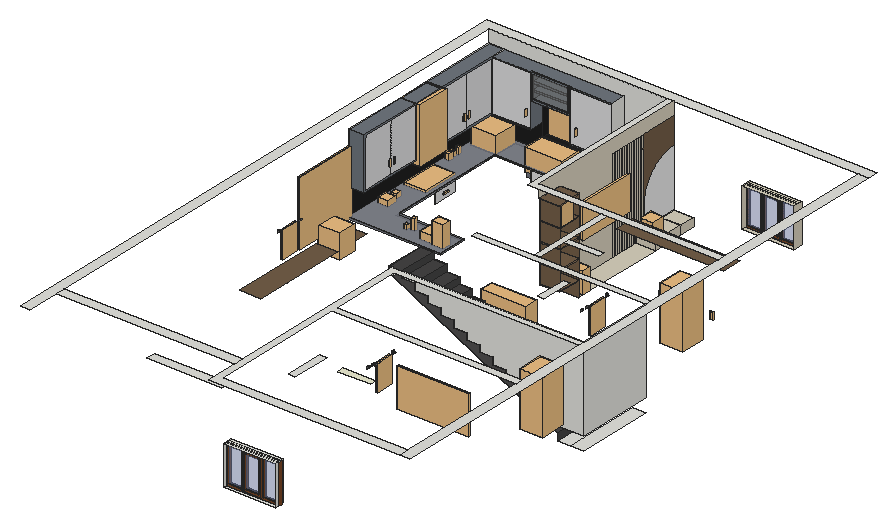
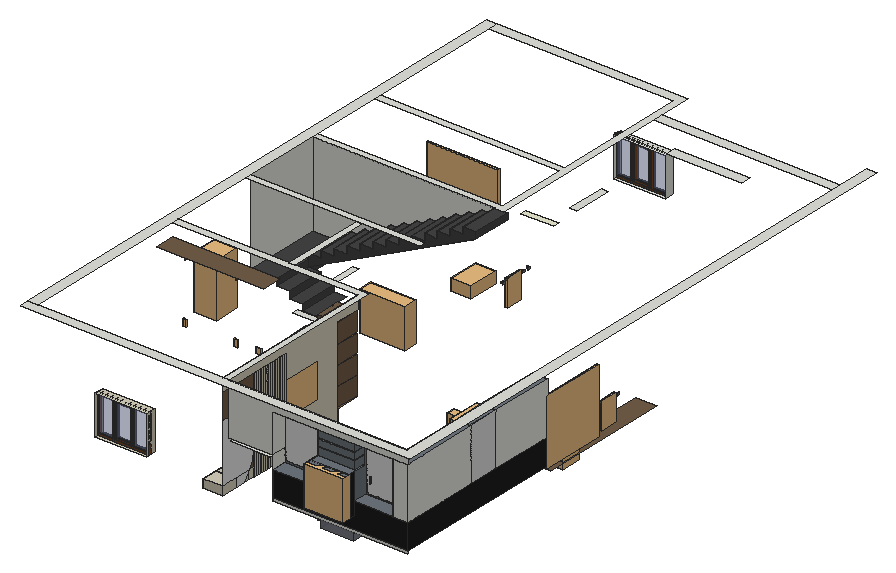
# SketchUp Ruby script. Lengths in inches.
U = 1.inch
M = Sketchup.active_model
def pt(a) = Geom::Point3d.new(a.map { |v| v * U })
def face(e, loops, mat)
  f = e.add_face(loops[0].map { |a| pt(a) })
  loops[1..].each { |l| e.add_face(l.map { |a| pt(a) }).erase! }
  f.material = f.back_material = mat if mat
  f
end
# faces: each face lists its corners as indices into pts; further lists are holes
def faces(e, pts, list, mat = nil) = list.each { |f| face(e, (f[0].is_a?(Array) ? f : [f]).map { |l| l.map { |i| pts[i] } }, mat) }
# xy, xz, yz: faces in a plane at the given z, y or x. An outline is a flat list of corners, or four numbers for a rectangle; further outlines are holes
def ring(l) = l.size == 4 ? [[l[0], l[1]], [l[2], l[1]], [l[2], l[3]], [l[0], l[3]]] : l.each_slice(2).to_a
def flat(e, list, mat, &to3) = list.each { |f| face(e, (f[0].is_a?(Array) ? f : [f]).map { |l| ring(l).map { |u, v| to3.(u, v) } }, mat) }
def xy(e, z, list, mat = nil) = flat(e, list, mat) { |x, y| [x, y, z] }
def xz(e, y, list, mat = nil) = flat(e, list, mat) { |x, z| [x, y, z] }
def yz(e, x, list, mat = nil) = flat(e, list, mat) { |y, z| [x, y, z] }
def lines(e, pts, list) = list.each { |a, b| e.add_line(pt(pts[a]), pt(pts[b])) }
# prism: a flat outline (further loops are holes) pulled along v
def prism(e, loops, v, mat = nil)
  f = face(e, loops, mat); d = Geom::Vector3d.new(v.map { |x| x * U })
  f.pushpull(f.normal.samedirection?(d) ? d.length : -d.length)
end
def box(e, o, s, mat = nil) = prism(e, [[o, [o[0] + s[0], o[1], o[2]], [o[0] + s[0], o[1] + s[1], o[2]], [o[0], o[1] + s[1], o[2]]]], [0, 0, s[2]], mat)
def at(x, y, z, deg = 0) = Geom::Transformation.translation(pt([x, y, z])) * Geom::Transformation.rotation(ORIGIN, Z_AXIS, deg.degrees)
def axes(o, x, y, z) = Geom::Transformation.new([*x, 0, *y, 0, *z, 0, *pt(o).to_a, 1])
def part(name) = M.definitions.add(name)
# library, detail: a bought-in or finely detailed component or shape, given as its bounding box
def library(name, o, s) = part(name).tap { |d| box(d.entities, o, s) }
def detail(e, o, s) = box(e.add_group.entities, o, s)
def put(e, d, t, mat = nil) = e.add_instance(d, t).tap { |i| i.material = mat if mat }
def group(e, t, mat = nil) = e.add_group.tap { |g| g.transformation = t; g.material = mat if mat }.entities
root = M.entities
M.materials.add("0746 AP 7715 LUMINOUS").color = [235, 235, 209]
M.materials.add("1442 AP K091 Frozen Zanskar-N").color = [220, 220, 221]
M.materials.add("1446 AP 8255 STONE PATH").color = [111, 118, 125]
M.materials.add("1689 AP 8482 GREY BUCK").color = [214, 207, 188]
M.materials.add("CROMADO1").color = [109, 109, 109]
M.materials.add("Granite Padang Light 150cm").color = [116, 119, 128]
M.materials["Granite Padang Light 150cm"].alpha = 0.92
M.materials.add("Tiles Marble Black 01 160cm").color = [32, 32, 32]
M.materials.add("Wood Pecan 33-21 150cm").color = [115, 94, 72]
M.materials.add("Wood Walnut 33-38 100cm").color = [48, 31, 12]
M.materials.add("[Granite Dark Gray]").color = [69, 68, 68]
M.materials.add("[Mirror 02]").color = [229, 229, 229]
M.materials.add("[Translucent Glass Gray]").color = [128, 128, 128]
M.materials["[Translucent Glass Gray]"].alpha = 0.5
M.materials.add("[Translucent Glass Sky Reflection]1").color = [126, 138, 183]
M.materials["[Translucent Glass Sky Reflection]1"].alpha = 0.52
M.materials.add("[Wood Veneer 01]").color = [120, 70, 37]
M.materials.add("w-001").color = [255, 255, 255]
c1 = library("1-VASEFLEURS CLC2",[-4.93,-4.36,0],[9.88,8.02,19.93])
c2 = library("3-EVIER M60 CLC2\#1",[-8.86,-8.86,-7.51],[17.72,19.62,22.02])
c3 = library("1-POIGNEE CLC2\#1",[-3.03,-0.375,0],[6.06,0.75,1.42])
c4 = library("1-POIGNEE CLC2\#2",[-3.03,-0.375,0],[6.06,0.75,1.42])
c5 = library("4",[-16.3,-15.81,0],[32.6,31.62,37.8])
c6 = library("4-EVIER M80 CLC2",[-16.92,-9.84,-5.67],[33.86,19.68,19.96])
c7 = library("Towel",[0,0,0],[10.6875,1.92,14.5625])
c8 = library("MOROCCAN+WASH+BASIN",[-11.85,-9.27,0.39],[28.27,18.54,10.92])
c9 = library("HUDSON+mirror",[-29.92,-0.89,23.77],[59.84,1.78,59.94])
c10 = library("1-MICRO H40 CLC2",[0,-1.46,0],[23.5,21.66,15.63])
c11 = library("1-PNGFRUITS CLC2",[-5.8,-5.64,-0.15],[11.3,11.71,6.42])
c12 = part("beroom window")
xy(c12.entities,-0.21,[[0,2.95,48.51,5.71]],"[Wood Veneer 01]")
xy(c12.entities,0.95,[[16.09,2.17,32.42,2.95]],"[Wood Veneer 01]")
xy(c12.entities,1.1875,[[1.44,2.95,14.41,4.33],[16.33,2.95,32.18,4.92],[34.1,2.95,47.07,4.33],[1.44,4.33,14.41,5.71],[34.1,4.33,47.07,5.71],
  [16.33,4.92,32.18,5.71]],"[Wood Veneer 01]")
xy(c12.entities,2.58,[[17.77,2.17,30.74,3.54],[17.77,3.54,30.74,4.92]],"[Wood Veneer 01]")
xy(c12.entities,29.62,[[17.77,2.17,30.74,3.54],[17.77,3.54,30.74,4.92]],"[Wood Veneer 01]")
xy(c12.entities,31.02,[[1.44,2.95,14.41,4.33],[16.33,2.95,32.18,4.92],[34.1,2.95,47.07,4.33],[1.44,4.33,14.41,5.71],[34.1,4.33,47.07,5.71],
  [16.33,4.92,32.18,5.71]],"[Wood Veneer 01]")
xy(c12.entities,31.25,[[16.09,2.17,32.42,2.95]],"[Wood Veneer 01]")
xy(c12.entities,32.42,[[0,2.95,48.51,5.71]],"[Wood Veneer 01]")
xz(c12.entities,2.17,[[[16.09,0.95,32.42,31.25],[17.77,2.58,30.74,29.62]]],"[Wood Veneer 01]")
xz(c12.entities,2.95,[[[0,-0.21,48.51,32.42],[16.33,1.1875,32.18,31.02],[1.44,1.1875,14.41,31.02],[34.1,1.1875,47.07,31.02]]],"[Wood Veneer 01]")
xz(c12.entities,3.54,[[17.77,2.58,30.74,29.62]],"[Translucent Glass Sky Reflection]1")
xz(c12.entities,4.33,[[1.44,1.1875,14.41,31.02],[34.1,1.1875,47.07,31.02]],"[Translucent Glass Sky Reflection]1")
xz(c12.entities,4.92,[[[16.33,1.1875,32.18,31.02],[17.77,2.58,30.74,29.62]]],"[Wood Veneer 01]")
xz(c12.entities,5.71,[[[0,-0.21,48.51,32.42],[16.33,1.1875,32.18,31.02],[1.44,1.1875,14.41,31.02],[34.1,1.1875,47.07,31.02]]],"[Wood Veneer 01]")
yz(c12.entities,0,[[2.95,-0.21,5.71,32.42]],"[Wood Veneer 01]")
yz(c12.entities,1.44,[[2.95,1.1875,4.33,31.02],[4.33,1.1875,5.71,31.02]],"[Wood Veneer 01]")
yz(c12.entities,14.41,[[2.95,1.1875,4.33,31.02],[4.33,1.1875,5.71,31.02]],"[Wood Veneer 01]")
yz(c12.entities,16.09,[[2.17,0.95,2.95,31.25]],"[Wood Veneer 01]")
yz(c12.entities,16.33,[[2.95,1.1875,4.92,31.02],[4.92,1.1875,5.71,31.02]],"[Wood Veneer 01]")
yz(c12.entities,17.77,[[2.17,2.58,3.54,29.62],[3.54,2.58,4.92,29.62]],"[Wood Veneer 01]")
yz(c12.entities,30.74,[[2.17,2.58,3.54,29.62],[3.54,2.58,4.92,29.62]],"[Wood Veneer 01]")
yz(c12.entities,32.18,[[2.95,1.1875,4.92,31.02],[4.92,1.1875,5.71,31.02]],"[Wood Veneer 01]")
yz(c12.entities,32.42,[[2.17,0.95,2.95,31.25]],"[Wood Veneer 01]")
yz(c12.entities,34.1,[[2.95,1.1875,4.33,31.02],[4.33,1.1875,5.71,31.02]],"[Wood Veneer 01]")
yz(c12.entities,47.07,[[2.95,1.1875,4.33,31.02],[4.33,1.1875,5.71,31.02]],"[Wood Veneer 01]")
yz(c12.entities,48.51,[[2.95,-0.21,5.71,32.42]],"[Wood Veneer 01]")
g1 = group(c12.entities,at(16.61,2.17,13.98),"w-001")
xy(g1,0,[[0.12,-2.17,0.53,-1.77]])
xy(g1,1.57,[[0,-0.39,0.65,0]])
xy(g1,2.1,[[0.12,-1.77,0.53,-0.39]])
xy(g1,2.5625,[[0.12,-2.17,0.53,-0.39]])
xy(g1,3.09,[[0,-0.39,0.65,0]])
xz(g1,-2.17,[[0.12,0,0.53,2.5625]])
xz(g1,-1.77,[[0.12,0,0.53,2.1]])
xz(g1,-0.39,[[[0,1.57,0.65,3.09],[0.12,2.1,0.53,2.5625]]])
xz(g1,0,[[0,1.57,0.65,3.09]])
yz(g1,0,[[-0.39,1.57,0,3.09]])
yz(g1,0.12,[[-2.17,0,-2.17,2.5625,-0.39,2.5625,-0.39,2.1,-1.77,2.1,-1.77,0]])
yz(g1,0.53,[[-2.17,0,-1.77,0,-1.77,2.1,-0.39,2.1,-0.39,2.5625,-2.17,2.5625]])
yz(g1,0.65,[[-0.39,1.57,0,3.09]])
c13 = library("16-PRODUITS CUISINE CLC2",[-2.49,-2.49,0],[4.98,4.98,4.3])
c14 = library("10-PRODUITS CUISINE CLC2",[-4.7,-4.62,0],[9.45,9.45,4.72])
c15 = library("3-PRODUITS CUISINE CLC2",[-1.54,-1.54,0],[3.08,3.08,10.36])
c16 = library("13-PRODUITS CUISINE CLC2",[-1.97,-1.97,0],[3.94,3.94,3.9375])
c17 = library("20-PRODUITS CUISINE CLC2",[-1.38,-1.38,0],[2.76,2.76,3.9375])
c18 = library("15-PRODUITS CUISINE CLC2",[-1.94,-2.15,0],[3.93,3.94,5.51])
c19 = library("22-PRODUITS CUISINE CLC2",[-2.93,-2.91,0],[5.9,5.9,2.76])
c20 = library("7-TABLE DE CUISSON CLC2",[-16.93,-10.04,0.13],[33.86,20.08,1.97])
c21 = library("23-PRODUITS CUISINE CLC2",[-4.92,-4.92,-0.18],[9.84,9.84,0.98])
c22 = library("11-PRODUITS CUISINE CLC2",[-1.48,-1.48,0],[2.96,2.96,6.14])
c23 = library("deca slim quadrada",[0,0,0],[0.79,5.12,5.12])
c24 = library("Bathroom vanity",[0,-2.21,0],[70.12,25.94,41.93])
c25 = library("Kitchen Window",[0,0,0],[58.5625,13.48,48])
c26 = library("Shower Raindance Connect",[1.71,-11.67,0],[20.76,23.22,49.85])
c27 = library("Ribe+Handles+timber",[52.85,54.46,0],[0.74,3.05,6.14])
c28 = library("Flat screen television",[-21.7,-0.05,0],[43.4,2.31,25.36])
c29 = part("Group\#170")
g2 = group(c29.entities,at(0.87,1.79,0.87))
box(g2,[-0.87,-0.39,-0.87],[1.74,0.39,1.74],"CROMADO1")
g3 = group(c29.entities,at(0.87,1.79,0.87))
prism(g3,[[[-0.1875,-1.42,1.39],[-0.1875,-1.42,0.1875],[-0.1875,-0.39,0.1875],[-0.1875,-0.39,-0.1875],[-0.1875,-1.79,-0.1875],[-0.1875,-1.79,1.39]]],[0.375,0,0],"CROMADO1")
c30 = part("Group\#166")
xy(c30.entities,0,[[-6.57,-0.87,-6.59,-0.85,-6.59,0.85,-6.57,0.87,-4.87,0.87,-4.85,0.85,-4.85,-0.85,-4.87,-0.87],[16.68,-0.87,16.66,-0.85,16.66,0.85,16.68,0.87,18.38,0.87,18.4,0.85,18.4,-0.85,18.38,-0.87]],"CROMADO1")
xy(c30.entities,0.39,[[[-6.57,-0.87,-4.87,-0.87,-4.85,-0.85,-4.85,0.85,-4.87,0.87,-6.57,0.87,-6.59,0.85,-6.59,-0.85],[-5.91,-0.1875,-5.53,0.1875]],[[16.68,-0.87,18.38,-0.87,18.4,-0.85,18.4,0.85,18.38,0.87,16.68,0.87,16.66,0.85,16.66,-0.85],[17.34,-0.1875,17.72,0.1875]]],"CROMADO1")
xy(c30.entities,2.15,[[-5.53,-0.1875,17.34,0.1875]],"CROMADO1")
xy(c30.entities,2.52,[[-5.91,-0.1875,17.72,0.1875]],"CROMADO1")
xz(c30.entities,-0.87,[[-6.57,0,-4.87,0.39],[16.68,0,18.38,0.39]],"CROMADO1")
xz(c30.entities,-0.1875,[[-5.91,0.39,-5.53,0.39,-5.53,2.15,17.34,2.15,17.34,0.39,17.72,0.39,17.72,2.52,-5.91,2.52]])
xz(c30.entities,0.1875,[[-5.91,0.39,-5.91,2.52,17.72,2.52,17.72,0.39,17.34,0.39,17.34,2.15,-5.53,2.15,-5.53,0.39]],"CROMADO1")
xz(c30.entities,0.87,[[-6.57,0,-4.87,0.39],[16.68,0,18.38,0.39]],"CROMADO1")
yz(c30.entities,-6.59,[[-0.85,0,0.85,0.39]],"CROMADO1")
yz(c30.entities,-5.91,[[-0.1875,0.39,0.1875,2.52]],"CROMADO1")
yz(c30.entities,-5.53,[[-0.1875,0.39,0.1875,2.15]],"CROMADO1")
yz(c30.entities,-4.85,[[-0.85,0,0.85,0.39]],"CROMADO1")
yz(c30.entities,16.66,[[-0.85,0,0.85,0.39]],"CROMADO1")
yz(c30.entities,17.34,[[-0.1875,0.39,0.1875,2.15]],"CROMADO1")
yz(c30.entities,17.72,[[-0.1875,0.39,0.1875,2.52]],"CROMADO1")
yz(c30.entities,18.4,[[-0.85,0,0.85,0.39]],"CROMADO1")
p = [[-6.57,-0.87,0.39],[-6.59,-0.85,0.39],[-6.59,-0.85,0],[-6.57,-0.87,0],[-4.85,-0.85,0.39],[-4.87,-0.87,0.39],
  [-4.87,-0.87,0],[-4.85,-0.85,0],[16.68,-0.87,0.39],[16.66,-0.85,0.39],[16.66,-0.85,0],[16.68,-0.87,0],
  [18.4,-0.85,0],[18.4,-0.85,0.39],[18.38,-0.87,0.39],[18.38,-0.87,0],[-6.57,0.87,0],[-6.59,0.85,0],
  [-6.59,0.85,0.39],[-6.57,0.87,0.39],[-4.85,0.85,0],[-4.87,0.87,0],[-4.87,0.87,0.39],[-4.85,0.85,0.39],
  [16.68,0.87,0.39],[16.68,0.87,0],[16.66,0.85,0],[16.66,0.85,0.39],[18.38,0.87,0],[18.38,0.87,0.39],
  [18.4,0.85,0.39],[18.4,0.85,0]]
faces(c30.entities,p,[[0,1,2,3],[4,5,6,7],[8,9,10,11],[12,13,14,15],[16,17,18,19],[20,21,22,23],[24,25,26,27],[28,29,30,31]])
c31 = library("5-HOTTE ASPIRANTE CLC2",[-15.16,-17.72,-0.29],[30.34,17.72,30.09])
c32 = library("Dekoracija24",[-23.93,-1.04,68.5625],[48.15,1.24,26.11])
c33 = library("1-POIGNEE CLC2\#3",[-3.03,-0.375,0],[6.06,0.75,1.42])
c34 = library("6-VASEFLEURS CLC2",[-8.63,-6.29,0],[14.28,12.79,17.02])
xy(root,22,[[180,399,198,487],[179.5,459,180,460],[179.5,461,180,462],[179.5,463,180,464],[179.5,465,180,466],
  [179.5,467,180,468],[179.5,469,180,470],[179.5,471,180,472],[179.5,473,180,474],[179.5,475,180,476],
  [179.5,477,180,478],[179.5,479,180,480],[179.5,481,180,482],[179.5,483,180,484],[179.5,485,180,486],
  [179.5,487,180,488],[180,487,198,495],[179.5,489,180,490],[179.5,491,180,492],[179.5,493,180,494],
  [180,495,198,501.67],[180,501.67,198,516.33],[180,516.33,198,531]],"1689 AP 8482 GREY BUCK")
xy(root,23.7,[[32.7,438.9,33,461.4],[66.97,507,100.33,507.3]],"1442 AP K091 Frozen Zanskar-N")
xy(root,24,[[32.7,438.9,32.8,461.4],[32.8,438.9,33,461.4],[66.97,507,100.33,507.3]],"1442 AP K091 Frozen Zanskar-N")
xy(root,24,[[61.45,509.36,92.2,527.24]],"Granite Padang Light 150cm")
xy(root,24,[[291,249,303,285]],"[Granite Dark Gray]")
xy(root,29,[[28.39,273.63,28.6875,273.93],[28.39,333.67,28.6875,333.97]],"Wood Pecan 33-21 150cm")
xy(root,30,[[327,213,339,249],[339,213,351,285]])
xy(root,30,[[180,487,198,501.67],[180,501.67,198,516.33],[180,516.33,198,531]],"1689 AP 8482 GREY BUCK")
xy(root,30,[[[9,242.61,28.6875,364.7],[19.02,331.45,16.86,331.97,14.9,333.03,13.29,334.5625,12.125,336.46,11.49,338.59,11.43,340.82,11.95,342.98,13.01,344.9375,14.55,346.55,16.44,347.71,18.58,348.35,20.8,348.4,22.96,347.88,24.92,346.82,26.53,345.29,27.7,343.39,28.33,341.26,28.39,339.04,27.87,336.87,26.81,334.92,25.27,333.3,23.375,332.14,21.24,331.51]]],"Wood Pecan 33-21 150cm")
xy(root,30,[[303,249,315,285]],"[Granite Dark Gray]")
xy(root,34,[[9,367,95,369],[93,369,95,393],[62.7,392.7,62.7,393,33,393,33,415.8,32.7,415.8,32.7,416.1,33,416.1,33,438.6,32.7,438.6,32.7,438.9,33,438.9,33,461.4,32.7,461.4,32.7,461.7,33,461.7,33,484.2,32.7,484.2,32.7,484.5,33,484.5,33,507,66.67,507,66.67,507.3,66.97,507.3,66.97,507,100.33,507,100.33,507.3,100.63,507.3,100.63,507,134,507,134,505,35,505,35,395,95,395,95,393,63,393,63,392.7]],"Granite Padang Light 150cm")
xy(root,36,[[188,0,236,9]])
xy(root,36,[[243,531,291,540]],"1689 AP 8482 GREY BUCK")
xy(root,36,[[[9,367,95,367,95,395,35,395,35,505,134,505,134,531,9,531],[61.45,509.36,92.2,527.24]]],"Granite Padang Light 150cm")
xy(root,36,[[180,376,198,398]],"Wood Pecan 33-21 150cm")
xy(root,36,[[315,249,327,285]],"[Granite Dark Gray]")
xy(root,37,[[180,376,198,398]],"Wood Pecan 33-21 150cm")
xy(root,42,[[327,213,351,285]],"[Granite Dark Gray]")
xy(root,48,[[58.6875,531,94.6875,540]],"Tiles Marble Black 01 160cm")
xy(root,48,[[315,213,327,249]],"[Granite Dark Gray]")
xy(root,53.5,[[180,376,198,398]],"Wood Pecan 33-21 150cm")
xy(root,54,[[303,213,315,249]],"[Granite Dark Gray]")
xy(root,54.5,[[180,376,198,398]],"Wood Pecan 33-21 150cm")
xy(root,60,[[9,369,23,428.6],[9,457.4,23,531],[23,517,58.6875,531],[94.6875,517,134,531]],"1446 AP 8255 STONE PATH")
xy(root,60,[[291,213,303,249]],"[Granite Dark Gray]")
xy(root,62,[[22.7,399.8,23,400.1],[22.7,486.2,23,486.5]])
xy(root,66,[[279,213,291,249]],"[Granite Dark Gray]")
xy(root,70,[[136,495,172,531]])
xy(root,71,[[180,376,198,398]],"Wood Pecan 33-21 150cm")
xy(root,72,[[188,0,236,9]])
xy(root,72,[[186,135,216,141]],"0746 AP 7715 LUMINOUS")
xy(root,72,[[243,531,291,540]],"1689 AP 8482 GREY BUCK")
xy(root,72,[[180,376,198,398]],"Wood Pecan 33-21 150cm")
xy(root,72,[[134,495,174,531]],"Wood Walnut 33-38 100cm")
xy(root,72,[[267,213,279,249]],"[Granite Dark Gray]")
xy(root,78,[[255,213,267,249]],"[Granite Dark Gray]")
xy(root,84,[[174,93,180,129],[243,295,248,325],[204,369,240,375]])
xy(root,84,[[58.6875,518,94.6875,540]],"1446 AP 8255 STONE PATH")
xy(root,84,[[243,213,255,249]],"[Granite Dark Gray]")
xy(root,85,[[59.6875,518,93.6875,529]],"1446 AP 8255 STONE PATH")
xy(root,88.5,[[180,376,198,398]],"Wood Pecan 33-21 150cm")
xy(root,89.5,[[180,376,198,398]],"Wood Pecan 33-21 150cm")
xy(root,90,[[231,213,243,249]],"[Granite Dark Gray]")
xy(root,92,[[59.6875,518,93.6875,529]],"1446 AP 8255 STONE PATH")
xy(root,93,[[59.6875,518,93.6875,529]],"1446 AP 8255 STONE PATH")
xy(root,96,[[92.875,30.5,162,39.5]])
xy(root,96,[[219,213,231,249]],"[Granite Dark Gray]")
xy(root,99,[[59.6875,518,93.6875,529]],"1446 AP 8255 STONE PATH")
xy(root,100,[[59.6875,518,93.6875,529]],"1446 AP 8255 STONE PATH")
xy(root,102,[[207,213,219,249]],"[Granite Dark Gray]")
xy(root,106,[[22.7,399.8,23,400.1],[22.7,486.2,23,486.5]])
xy(root,106,[[277.45,392.7,277.75,393],[324.95,392.7,325.25,393]],"1689 AP 8482 GREY BUCK")
xy(root,107,[[59.6875,518,93.6875,529]],"1446 AP 8255 STONE PATH")
xy(root,107,[[180,376,198,398]],"Wood Pecan 33-21 150cm")
xy(root,108,[[9,369,23,428.6],[9,428.6,23,457.4],[9,457.4,23,531],[23,517,58.6875,517,58.6875,518,94.6875,518,94.6875,517,134,517,134,531,23,531]],"1446 AP 8255 STONE PATH")
xy(root,108,[[179.5,459,180,460],[179.5,461,180,462],[179.5,463,180,464],[179.5,465,180,466],[179.5,467,180,468],
  [179.5,469,180,470],[179.5,471,180,472],[179.5,473,180,474],[179.5,475,180,476],[179.5,477,180,478],
  [179.5,479,180,480],[179.5,481,180,482],[179.5,483,180,484],[179.5,485,180,486],[179.5,487,180,488],
  [179.5,489,180,490],[179.5,491,180,492],[179.5,493,180,494]],"1689 AP 8482 GREY BUCK")
xy(root,108,[[180,375,198,399],[252,375,351,393]],"Wood Pecan 33-21 150cm")
xy(root,108,[[195,213,207,249]],"[Granite Dark Gray]")
xy(root,114,[[183,213,195,249]],"[Granite Dark Gray]")
xy(root,120,[[0,0,9,0,9,531,360,531,360,540,0,540],[174,0,351,0,351,9,180,9,180,135,351,135,351,141,180,141,180,207,351,207,351,213,174,213],[351,0,360,531],[9,30.5,174,39.5],[189.8125,285,351,291],
  [243,291,248,369],[174,369,351,369,351,375,180,375,180,531,174,531]])
xy(root,120,[[171,213,183,249]],"[Granite Dark Gray]")
xz(root,213,[[327,42,327,48,315,48,315,54,303,54,303,60,291,60,291,66,279,66,279,72,267,72,267,78,255,78,255,84,243,84,243,90,231,90,231,96,219,96,219,102,207,102,207,108,195,108,195,114,183,114,183,120,351,120,351,42],[174,112.5,174,120,171,120,171,114]])
xz(root,249,[[327,36,171,114,171,120,183,120,183,114,195,114,195,108,207,108,207,102,219,102,219,96,231,96,231,90,243,90,243,84,255,84,255,78,267,78,267,72,279,72,279,66,291,66,291,60,303,60,303,54,315,54,315,48,327,48]],"[Granite Dark Gray]")
xz(root,367,[[9,34,95,36]],"Granite Padang Light 150cm")
xz(root,369,[[9,60,23,108]],"1446 AP 8255 STONE PATH")
xz(root,376,[[180,37,198,53.5],[180,54.5,198,71],[180,72,198,88.5],[180,89.5,198,107]],"Wood Pecan 33-21 150cm")
xz(root,395,[[35,34,95,36]],"Granite Padang Light 150cm")
xz(root,398,[[180,22,198,36],[180,37,198,53.5],[180,54.5,198,71],[180,72,198,88.5],[180,89.5,198,107]],"Wood Pecan 33-21 150cm")
xz(root,399,[[180,22,198,108]],"Wood Pecan 33-21 150cm")
xz(root,399.8,[[22.7,62,23,106]],"1442 AP K091 Frozen Zanskar-N")
xz(root,400.1,[[22.7,62,23,106]],"1442 AP K091 Frozen Zanskar-N")
xz(root,428.6,[[9,60,23,108]],"1446 AP 8255 STONE PATH")
xz(root,438.9,[[32.7,24,33,34]],"1442 AP K091 Frozen Zanskar-N")
xz(root,457.4,[[9,60,23,106],[9,106,23,108]],"1446 AP 8255 STONE PATH")
xz(root,459,[[179.5,22,180,108]],"1689 AP 8482 GREY BUCK")
xz(root,460,[[179.5,22,180,108]],"1689 AP 8482 GREY BUCK")
xz(root,461,[[179.5,22,180,108]],"1689 AP 8482 GREY BUCK")
xz(root,461.4,[[32.7,24,33,34]],"1442 AP K091 Frozen Zanskar-N")
xz(root,462,[[179.5,22,180,108]],"1689 AP 8482 GREY BUCK")
xz(root,463,[[179.5,22,180,108]],"1689 AP 8482 GREY BUCK")
xz(root,464,[[179.5,22,180,108]],"1689 AP 8482 GREY BUCK")
xz(root,465,[[179.5,22,180,108]],"1689 AP 8482 GREY BUCK")
xz(root,466,[[179.5,22,180,108]],"1689 AP 8482 GREY BUCK")
xz(root,467,[[179.5,22,180,108]],"1689 AP 8482 GREY BUCK")
xz(root,468,[[179.5,22,180,108]],"1689 AP 8482 GREY BUCK")
xz(root,469,[[179.5,22,180,108]],"1689 AP 8482 GREY BUCK")
xz(root,470,[[179.5,22,180,108]],"1689 AP 8482 GREY BUCK")
xz(root,471,[[179.5,22,180,108]],"1689 AP 8482 GREY BUCK")
xz(root,472,[[179.5,22,180,108]],"1689 AP 8482 GREY BUCK")
xz(root,473,[[179.5,22,180,108]],"1689 AP 8482 GREY BUCK")
xz(root,474,[[179.5,22,180,108]],"1689 AP 8482 GREY BUCK")
xz(root,475,[[179.5,22,180,108]],"1689 AP 8482 GREY BUCK")
xz(root,476,[[179.5,22,180,108]],"1689 AP 8482 GREY BUCK")
xz(root,477,[[179.5,22,180,108]],"1689 AP 8482 GREY BUCK")
xz(root,478,[[179.5,22,180,108]],"1689 AP 8482 GREY BUCK")
xz(root,479,[[179.5,22,180,108]],"1689 AP 8482 GREY BUCK")
xz(root,480,[[179.5,22,180,108]],"1689 AP 8482 GREY BUCK")
xz(root,481,[[179.5,22,180,108]],"1689 AP 8482 GREY BUCK")
xz(root,482,[[179.5,22,180,108]],"1689 AP 8482 GREY BUCK")
xz(root,483,[[179.5,22,180,108]],"1689 AP 8482 GREY BUCK")
xz(root,484,[[179.5,22,180,108]],"1689 AP 8482 GREY BUCK")
xz(root,485,[[179.5,22,180,108]],"1689 AP 8482 GREY BUCK")
xz(root,486,[[179.5,22,180,108]],"1689 AP 8482 GREY BUCK")
xz(root,486.2,[[22.7,62,23,106]],"1442 AP K091 Frozen Zanskar-N")
xz(root,486.5,[[22.7,62,23,106]],"1442 AP K091 Frozen Zanskar-N")
xz(root,487,[[179.5,22,180,108],[180,22,198,30]],"1689 AP 8482 GREY BUCK")
xz(root,488,[[179.5,22,180,108]],"1689 AP 8482 GREY BUCK")
xz(root,489,[[179.5,22,180,108]],"1689 AP 8482 GREY BUCK")
xz(root,490,[[179.5,22,180,108]],"1689 AP 8482 GREY BUCK")
xz(root,491,[[179.5,22,180,108]],"1689 AP 8482 GREY BUCK")
xz(root,492,[[179.5,22,180,108]],"1689 AP 8482 GREY BUCK")
xz(root,493,[[179.5,22,180,108]],"1689 AP 8482 GREY BUCK")
xz(root,494,[[179.5,22,180,108]],"1689 AP 8482 GREY BUCK")
xz(root,501.67,[[180,22,198,30]],"1689 AP 8482 GREY BUCK")
xz(root,505,[[35,34,134,36]],"Granite Padang Light 150cm")
xz(root,507,[[66.97,24,100.33,34]],"1442 AP K091 Frozen Zanskar-N")
xz(root,507.3,[[66.97,23.7,100.33,24]],"1442 AP K091 Frozen Zanskar-N")
xz(root,509.36,[[61.45,24,92.2,36]],"Granite Padang Light 150cm")
xz(root,516.33,[[180,22,198,30]],"1689 AP 8482 GREY BUCK")
xz(root,517,[[24,61,57.6875,107],[95.6875,61,133,107]],"1442 AP K091 Frozen Zanskar-N")
xz(root,517,[[[23,60,58.6875,108],[24,61,57.6875,107]],[[94.6875,60,134,108],[95.6875,61,133,107]]],"1446 AP 8255 STONE PATH")
xz(root,518,[[[58.6875,84,94.6875,108],[59.6875,100,93.6875,107],[59.6875,85,93.6875,92],[59.6875,93,93.6875,99]]],"1446 AP 8255 STONE PATH")
xz(root,527.24,[[61.45,24,92.2,36]],"Granite Padang Light 150cm")
xz(root,529,[[59.6875,85,93.6875,92],[59.6875,93,93.6875,99],[59.6875,100,93.6875,107]],"1446 AP 8255 STONE PATH")
xz(root,531,[[9,34,134,36],[9,60,23,108],[134,72,174,72,174,120,9,120,9,108,134,108]])
xz(root,531,[[180,22,198,30]],"1689 AP 8482 GREY BUCK")
xz(root,531,[[9,36,134,36,134,60,94.6875,60,94.6875,48,58.6875,48,58.6875,60,9,60]],"Tiles Marble Black 01 160cm")
yz(root,9,[[369,60,428.6,108],[457.4,60,531,108]])
yz(root,9,[[428.6,60,457.4,108]],"1442 AP K091 Frozen Zanskar-N")
yz(root,9,[[369,36,531,60]],"Tiles Marble Black 01 160cm")
yz(root,22.7,[[399.8,62,400.1,106],[486.2,62,486.5,106]],"1442 AP K091 Frozen Zanskar-N")
yz(root,23,[[517,60,531,108]])
yz(root,23,[[371,62,399.8,106],[400.1,62,427.6,106],[458.4,62,486.2,106],[486.5,62,515,106],[429.6,89.89,456.4,107]],"1442 AP K091 Frozen Zanskar-N")
yz(root,23,[[[369,60,428.6,108],[371,62,427.6,106]],[[457.4,60,517,108],[458.4,62,515,106]],[[428.6,88.89,457.4,108],[429.6,89.89,456.4,107]]],"1446 AP 8255 STONE PATH")
yz(root,32.7,[[438.9,23.7,461.4,24]],"1442 AP K091 Frozen Zanskar-N")
yz(root,33,[[438.9,24,461.4,34]],"1442 AP K091 Frozen Zanskar-N")
yz(root,35,[[395,34,505,36]],"Granite Padang Light 150cm")
yz(root,58.6875,[[517,60,531,60,531,84,518,84,518,108,517,108]],"1446 AP 8255 STONE PATH")
yz(root,58.6875,[[531,48,540,84]],"Tiles Marble Black 01 160cm")
yz(root,59.6875,[[518,85,529,92],[518,93,529,99],[518,100,529,107]],"1446 AP 8255 STONE PATH")
yz(root,61.45,[[509.36,24,527.24,36]],"Granite Padang Light 150cm")
yz(root,66.97,[[507,24,507.3,34]])
yz(root,92.2,[[509.36,24,527.24,36]],"Granite Padang Light 150cm")
yz(root,93.6875,[[518,85,529,92],[518,93,529,99],[518,100,529,107]],"1446 AP 8255 STONE PATH")
yz(root,94.6875,[[517,60,517,108,518,108,518,84,531,84,531,60]])
yz(root,94.6875,[[531,48,540,84]],"Tiles Marble Black 01 160cm")
yz(root,95,[[367,34,395,36]],"Granite Padang Light 150cm")
yz(root,100.33,[[507,24,507.3,34]])
yz(root,134,[[505,34,531,36],[517,60,531,72],[517,72,531,108]])
yz(root,134,[[495,36,495,72,517,72,517,60,531,60,531,36]],"Wood Walnut 33-38 100cm")
yz(root,171,[[213,114,249,120]],"[Granite Dark Gray]")
yz(root,179.5,[[459,22,460,108],[461,22,462,108],[463,22,464,108],[465,22,466,108],[467,22,468,108],
  [469,22,470,108],[471,22,472,108],[473,22,474,108],[475,22,476,108],[477,22,478,108],
  [479,22,480,108],[481,22,482,108],[483,22,484,108],[485,22,486,108],[487,22,488,108],
  [489,22,490,108],[491,22,492,108],[493,22,494,108]],"1689 AP 8482 GREY BUCK")
yz(root,180,[[399,22,459,22,459,108,531,108,531,120,375,120,375,108,399,108],[460,22,461,108],[462,22,463,108],[464,22,465,108],[466,22,467,108],
  [468,22,469,108],[470,22,471,108],[472,22,473,108],[474,22,475,108],[476,22,477,108],
  [478,22,479,108],[480,22,481,108],[482,22,483,108],[484,22,485,108],[486,22,487,108],
  [487,22,488,30],[488,22,489,30],[489,22,490,30],[490,22,491,30],[491,22,492,30],
  [492,22,493,30],[493,22,494,30],[494,22,495,30],[495,22,495,30,500.51,30,501.03,29.13,501.67,28.13,501.67,22],[501.67,22,501.67,28.13,501.7,28.08,502.4,27.0625,503.14,26.0625,503.91,25.09,504.72,24.15,505.56,23.23,506.43,22.35,506.79,22],
  [516.33,22,531,30],[488,30,489,108],[490,30,491,108],[492,30,493,108],[494,30,495,108]],"1689 AP 8482 GREY BUCK")
yz(root,180,[[495,30,500.51,30,500.4,30.2,499.8,31.29,499.24,32.4,498.73,33.52,498.25,34.67,497.81,35.83,497.41,37.01,497.05,38.19,496.73,39.39,496.46,40.6,496.22,41.82,496.03,43.05,495.88,44.28,495.77,45.52,495.71,46.76,495.6875,48,495.71,49.24,495.77,50.48,495.88,51.72,496.03,52.95,496.22,54.18,496.46,55.4,496.73,56.61,497.05,57.81,497.41,58.99,497.81,60.17,498.25,61.33,498.73,62.48,499.24,63.6,499.8,64.71,500.4,65.8,501.03,66.87,501.7,67.92,502.4,68.9375,503.14,69.9375,503.91,70.91,504.72,71.85,505.56,72.77,506.43,73.65,507.33,74.51,508.26,75.33,509.21,76.125,510.19,76.88,511.2,77.61,512.24,78.3,513.29,78.95,514.37,79.56,515.47,80.14,516.59,80.68,517.72,81.18,518.875,81.65,520.04,82.07,521.22,82.45,522.42,82.79,523.62,83.09,524.83,83.35,526.06,83.5625,527.29,83.74,528.52,83.87,529.76,83.95,531,84,531,108,495,108],[376,37,398,53.5],[376,54.5,398,71],[376,72,398,88.5],[376,89.5,398,107]],"Wood Pecan 33-21 150cm")
yz(root,180,[[506.79,22,506.43,22.35,505.56,23.23,504.72,24.15,503.91,25.09,503.14,26.0625,502.4,27.0625,501.7,28.08,501.67,28.13,501.67,30,516.33,30,516.33,22],[501.67,28.13,501.03,29.13,500.51,30,501.67,30],[500.51,30,531,30,531,84,529.76,83.95,528.52,83.87,527.29,83.74,526.06,83.5625,524.83,83.35,523.62,83.09,522.42,82.79,521.22,82.45,520.04,82.07,518.875,81.65,517.72,81.18,516.59,80.68,515.47,80.14,514.37,79.56,513.29,78.95,512.24,78.3,511.2,77.61,510.19,76.88,509.21,76.125,508.26,75.33,507.33,74.51,506.43,73.65,505.56,72.77,504.72,71.85,503.91,70.91,503.14,69.9375,502.4,68.9375,501.7,67.92,501.03,66.87,500.4,65.8,499.8,64.71,499.24,63.6,498.73,62.48,498.25,61.33,497.81,60.17,497.41,58.99,497.05,57.81,496.73,56.61,496.46,55.4,496.22,54.18,496.03,52.95,495.88,51.72,495.77,50.48,495.71,49.24,495.6875,48,495.71,46.76,495.77,45.52,495.88,44.28,496.03,43.05,496.22,41.82,496.46,40.6,496.73,39.39,497.05,38.19,497.41,37.01,497.81,35.83,498.25,34.67,498.73,33.52,499.24,32.4,499.8,31.29,500.4,30.2]],"[Mirror 02]")
yz(root,183,[[213,114,249,120]],"[Granite Dark Gray]")
yz(root,188,[[0,36,9,72]])
yz(root,195,[[213,108,249,114]],"[Granite Dark Gray]")
yz(root,198,[[487,22,501.67,30],[501.67,22,516.33,30],[516.33,22,531,30]],"1689 AP 8482 GREY BUCK")
yz(root,207,[[213,102,249,108]],"[Granite Dark Gray]")
yz(root,219,[[213,96,249,102]],"[Granite Dark Gray]")
yz(root,231,[[213,90,249,96]],"[Granite Dark Gray]")
yz(root,236,[[0,36,9,72]])
yz(root,243,[[531,36,540,72]],"1689 AP 8482 GREY BUCK")
yz(root,243,[[213,84,249,90]],"[Granite Dark Gray]")
yz(root,255,[[213,78,249,84]],"[Granite Dark Gray]")
yz(root,267,[[213,72,249,78]],"[Granite Dark Gray]")
yz(root,279,[[213,66,249,72]],"[Granite Dark Gray]")
yz(root,291,[[531,36,540,72]],"1689 AP 8482 GREY BUCK")
yz(root,291,[[213,60,249,66]],"[Granite Dark Gray]")
yz(root,303,[[249,24,285,30],[213,54,249,60]],"[Granite Dark Gray]")
yz(root,315,[[249,30,285,36],[213,48,249,54]],"[Granite Dark Gray]")
yz(root,327,[[213,30,213,36,249,36,249,42,285,42,285,36,249,36,249,30],[213,42,249,48]],"[Granite Dark Gray]")
yz(root,351,[[213,42,285,120]])
p = [[327,213,36],[174,213,112.5],[174,249,112.5],[327,249,36],[171,213,114],[171,249,114],
  [32.7,438.9,34],[32.7,461.4,34]]
faces(root,p,[[0,1,2,3]],"[Granite Dark Gray]")
faces(root,p,[[1,4,5,2]])
lines(root,p,[[6,7]])
put(root,c1,at(192.99,407.61,22))
put(root,c2,at(21.24,340.3,30.97,90))
put(root,c3,axes([33,449.67,28.67],[0,1,0],[0,0,1],[1,0,0]))
put(root,c4,axes([83.73,507,29.15],[1,0,0],[0,0,1],[0,-1,0]))
put(root,c5,axes([188.95,494.1875,29.57],[0.3657,0,0],[0,0.3657,0],[0,0,0.3657]))
put(root,c6,at(77.8,517.34,36))
put(root,c7,axes([251.27,346,31.96],[0,1.5,0],[-1,0,0],[0,0,1.6614]))
put(root,c7,axes([183.27,184,31.96],[0,1.5,0],[-1,0,0],[0,0,1.6614]))
put(root,c8,at(218.67,195.21,32.04,-90))
put(root,c9,at(9.61,340.28,10.29,90))
put(root,c10,at(11.16,508.25,35))
put(root,c11,at(75.45,380.34,36))
put(root,c12,axes([188.19,0.32,36.23],[1,0,0],[0,1,0],[0,0,1.10328]))
put(root,c12,axes([243,532.32,36.23],[0.98945,0,0],[0,0.83,0],[0,0,1.10328]))
put(root,c1,at(86.91,377.75,36))
put(root,c13,at(17.41,412.59,36))
put(root,c14,at(17.83,401.65,36))
put(root,c15,at(58.375,382.36,36))
put(root,c16,at(11.88,484.71,36))
put(root,c17,at(52.91,380.77,36))
put(root,c18,at(12.59,479.73,36))
put(root,c19,at(116.16,514.59,36))
put(root,c20,at(21.43,446.6,36,90))
put(root,c21,at(106.92,520.86,36.4375))
put(root,c7,axes([12.27,288.75,36.32],[0,1.5,0],[-1,0,0],[0,0,1.6614]))
put(root,c22,at(14.01,488.98,36.8))
put(root,c23,at(276.1,371.84,36.8,90))
put(root,c21,at(108.1,520.57,37.38))
put(root,c24,axes([235.13,302.56,37.68],[-0.6,0,0],[0,-0.4872,0],[0,0,0.87]))
put(root,c25,axes([94.6875,543.89,48],[-0.61899,0,0],[0,-0.5607,0],[0,0,0.75]))
put(root,c26,at(313.62,357.45,48.49))
put(root,c26,at(313.62,195.45,48.49))
put(root,c27,at(381.125,340.15,50.91,90),"Wood Pecan 33-21 150cm")
put(root,c27,at(333.625,340.15,50.91,90),"Wood Pecan 33-21 150cm")
put(root,c28,axes([182.8,449,53.42],[0,1.24,0],[-1.24,0,0],[0,0,1.24]))
put(root,c29,at(249.79,337.76,54.24,90),"CROMADO1")
put(root,c29,at(181.79,175.76,54.24,90),"CROMADO1")
put(root,c30,axes([248,350.25,55.12],[0,1,0],[0,0,1],[1,0,0]),"CROMADO1")
put(root,c30,axes([180,188.25,55.12],[0,1,0],[0,0,1],[1,0,0]),"CROMADO1")
put(root,c31,axes([9.54,443.66,57.84],[0,0.99919,0],[-1,0,0],[0,0,1.68306]))
put(root,c30,axes([9,292.99,59.48],[0,1,0],[0,0,1],[1,0,0]),"CROMADO1")
put(root,c32,axes([274.59,134.93,-32.81],[1.37,0,0],[0,1.37,0],[0,0,1.37]))
put(root,c33,axes([100.63,517,72.62],[0,0,-1],[1,0,0],[0,-1,0]))
put(root,c33,axes([54.32,517,72.62],[0,0,-1],[1,0,0],[0,-1,0]))
put(root,c3,axes([23,402.59,72.75],[0,0,1],[0,-1,0],[1,0,0]))
put(root,c3,axes([23,397.47,72.75],[0,0,1],[0,-1,0],[1,0,0]))
put(root,c3,axes([23,483.87,72.75],[0,0,1],[0,-1,0],[1,0,0]))
put(root,c3,axes([23,488.99,72.75],[0,0,1],[0,-1,0],[1,0,0]))
g4 = group(root,at(58.6875,517,84))
xy(g4,0,[[0,0,36,1]],"1446 AP 8255 STONE PATH")
xy(g4,1.5,[[1.5,0,34.5,0.5],[1.5,0.5,34.5,1]],"1446 AP 8255 STONE PATH")
xy(g4,22.5,[[1.5,0,34.5,0.5],[1.5,0.5,34.5,1]],"1446 AP 8255 STONE PATH")
xy(g4,24,[[0,0,36,1]],"1446 AP 8255 STONE PATH")
xz(g4,0,[[[0,0,36,24],[1.5,1.5,34.5,22.5]]],"1446 AP 8255 STONE PATH")
xz(g4,0.5,[[1.5,1.5,34.5,22.5]],"[Translucent Glass Gray]")
xz(g4,1,[[[0,0,36,24],[1.5,1.5,34.5,22.5]]],"1446 AP 8255 STONE PATH")
yz(g4,0,[[0,0,1,24]],"1446 AP 8255 STONE PATH")
yz(g4,1.5,[[0,1.5,0.5,22.5],[0.5,1.5,1,22.5]],"1446 AP 8255 STONE PATH")
yz(g4,34.5,[[0,1.5,0.5,22.5],[0.5,1.5,1,22.5]],"1446 AP 8255 STONE PATH")
yz(g4,36,[[0,0,1,24]],"1446 AP 8255 STONE PATH")
put(root,c34,at(192.25,384.63,89.48))
